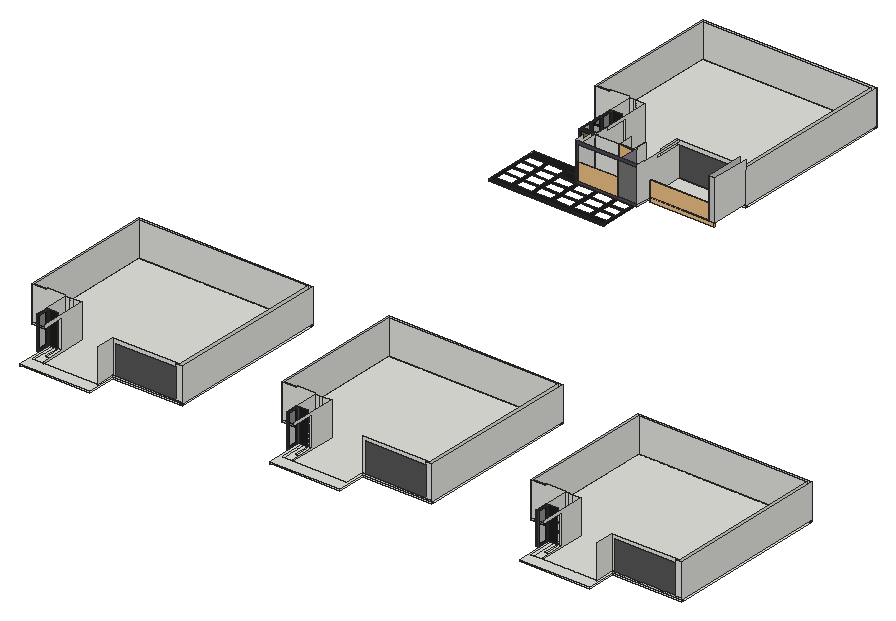
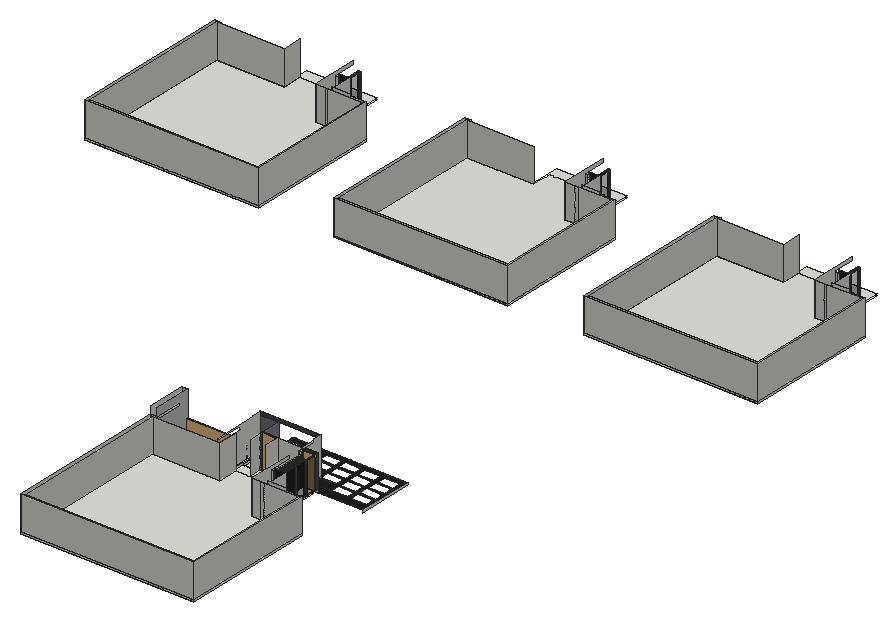
# SketchUp Ruby script. Lengths in inches.
U = 1.inch
M = Sketchup.active_model
def pt(a) = Geom::Point3d.new(a.map { |v| v * U })
def face(e, loops, mat)
  f = e.add_face(loops[0].map { |a| pt(a) })
  loops[1..].each { |l| e.add_face(l.map { |a| pt(a) }).erase! }
  f.material = f.back_material = mat if mat
  f
end
# faces: each face lists its corners as indices into pts; further lists are holes
def faces(e, pts, list, mat = nil) = list.each { |f| face(e, (f[0].is_a?(Array) ? f : [f]).map { |l| l.map { |i| pts[i] } }, mat) }
# xy, xz, yz: faces in a plane at the given z, y or x. An outline is a flat list of corners, or four numbers for a rectangle; further outlines are holes
def ring(l) = l.size == 4 ? [[l[0], l[1]], [l[2], l[1]], [l[2], l[3]], [l[0], l[3]]] : l.each_slice(2).to_a
def flat(e, list, mat, &to3) = list.each { |f| face(e, (f[0].is_a?(Array) ? f : [f]).map { |l| ring(l).map { |u, v| to3.(u, v) } }, mat) }
def xy(e, z, list, mat = nil) = flat(e, list, mat) { |x, y| [x, y, z] }
def xz(e, y, list, mat = nil) = flat(e, list, mat) { |x, z| [x, y, z] }
def yz(e, x, list, mat = nil) = flat(e, list, mat) { |y, z| [x, y, z] }
def lines(e, pts, list) = list.each { |a, b| e.add_line(pt(pts[a]), pt(pts[b])) }
# prism: a flat outline (further loops are holes) pulled along v
def prism(e, loops, v, mat = nil)
  f = face(e, loops, mat); d = Geom::Vector3d.new(v.map { |x| x * U })
  f.pushpull(f.normal.samedirection?(d) ? d.length : -d.length)
end
def box(e, o, s, mat = nil) = prism(e, [[o, [o[0] + s[0], o[1], o[2]], [o[0] + s[0], o[1] + s[1], o[2]], [o[0], o[1] + s[1], o[2]]]], [0, 0, s[2]], mat)
def at(x, y, z, deg = 0) = Geom::Transformation.translation(pt([x, y, z])) * Geom::Transformation.rotation(ORIGIN, Z_AXIS, deg.degrees)
def axes(o, x, y, z) = Geom::Transformation.new([*x, 0, *y, 0, *z, 0, *pt(o).to_a, 1])
def part(name) = M.definitions.add(name)
# library, detail: a bought-in or finely detailed component or shape, given as its bounding box
def library(name, o, s) = part(name).tap { |d| box(d.entities, o, s) }
def detail(e, o, s) = box(e.add_group.entities, o, s)
def put(e, d, t, mat = nil) = e.add_instance(d, t).tap { |i| i.material = mat if mat }
def group(e, t, mat = nil) = e.add_group.tap { |g| g.transformation = t; g.material = mat if mat }.entities
root = M.entities
M.materials.add("Glass_Tinted_Gray").color = [0, 0, 0]
M.materials["Glass_Tinted_Gray"].alpha = 0.125
M.materials.add("[0135_DarkGray]").color = [81, 81, 81]
M.materials.add("[Color M02]").color = [198, 198, 198]
M.materials.add("[Color M04]").color = [60, 133, 34]
M.materials.add("[Color M05]1").color = [114, 114, 114]
M.materials.add("[Color M06]").color = [79, 71, 84]
M.materials.add("[Color M06]1").color = [86, 86, 86]
M.materials.add("[Color M07]").color = [58, 58, 58]
M.materials.add("[Color M08]").color = [30, 30, 30]
M.materials.add("[Formica Graystone]1").color = [140, 132, 147]
M.materials.add("[Mirror 02]").color = [229, 229, 229]
c1 = part("PENTEK_RP Fineline 50S_SlidingDoor_Glass")
box(c1.entities,[0,0,0],[46.58,0.16,94.39],"Glass_Tinted_Gray")
c2 = part("PENTEK_RP Fineline 50S_SlidingDoor_GlazingBead")
box(c2.entities,[0,0,0],[45.47,0.59,0.56],"[0135_DarkGray]")
c3 = part("PENTEK_RP Fineline 50S_SlidingDoor_GlazingBead_2")
box(c3.entities,[0,0,0],[0.56,0.59,94.39],"[0135_DarkGray]")
c4 = part("PENTEK_RP Fineline 50S_SlidingDoor_Leaf_E1")
xy(c4.entities,0,[[0,0,0.93,1.97],[0.93,1.57,1.49,1.97]],"[0135_DarkGray]")
xy(c4.entities,96.25,[[0,0,0.93,0,0.93,1.57,1.49,1.57,1.49,1.97,0,1.97]],"[0135_DarkGray]")
xz(c4.entities,0,[[0,0,0.93,96.25]],"[0135_DarkGray]")
xz(c4.entities,1.57,[[0.93,0,1.49,95.32],[0.93,95.32,1.49,96.25]],"[0135_DarkGray]")
xz(c4.entities,1.97,[[0,0,1.49,96.25]],"[0135_DarkGray]")
yz(c4.entities,0,[[0,0,1.97,96.25]],"[0135_DarkGray]")
yz(c4.entities,0.93,[[0,0,1.57,0.93],[0,0.93,1.57,95.32],[0,95.32,1.57,96.25]],"[0135_DarkGray]")
yz(c4.entities,1.49,[[1.57,0,1.97,95.32],[1.57,95.32,1.97,96.25]],"[0135_DarkGray]")
c5 = part("PENTEK_RP Fineline 50S_SlidingDoor_Leaf_E2")
xy(c5.entities,0,[[0,0,0,1.57,0.56,1.57,0.56,1.97,46.02,1.97,46.02,1.57,46.58,1.57,46.58,0]],"[0135_DarkGray]")
xy(c5.entities,0.93,[[0,0,46.58,1.57]],"[0135_DarkGray]")
xy(c5.entities,1.49,[[0.56,1.57,46.02,1.97]],"[0135_DarkGray]")
xz(c5.entities,0,[[0,0,46.58,0.93]],"[0135_DarkGray]")
xz(c5.entities,1.57,[[0,0,0.56,0.93],[46.02,0,46.58,0.93],[0.56,0.93,46.02,1.49]],"[0135_DarkGray]")
xz(c5.entities,1.97,[[0.56,0,46.02,1.49]],"[0135_DarkGray]")
yz(c5.entities,0,[[0,0,1.57,0.93]],"[0135_DarkGray]")
yz(c5.entities,0.56,[[1.57,0,1.97,0.93],[1.57,0.93,1.97,1.49]],"[0135_DarkGray]")
yz(c5.entities,46.02,[[1.57,0,1.97,0.93],[1.57,0.93,1.97,1.49]],"[0135_DarkGray]")
yz(c5.entities,46.58,[[0,0,1.57,0.93]],"[0135_DarkGray]")
c6 = part("PENTEK_RP Fineline 50S_SlidingDoor_Leaf2")
put(c6.entities,c1,at(1.49,1.42,0.93))
put(c6.entities,c2,at(1.49,0,94.77))
put(c6.entities,c3,at(46.96,0,0.93))
put(c6.entities,c1,at(1.49,0.59,0.93),"[Mirror 02]")
put(c6.entities,c3,at(0.93,0,0.93))
put(c6.entities,c4,at(0,0,0))
put(c6.entities,c4,axes([48.44,0,0],[-1,0,0],[0,1,0],[0,0,1]))
put(c6.entities,c2,at(1.49,0,0.93))
put(c6.entities,c5,axes([0.93,0,96.25],[1,0,0],[0,1,0],[0,0,-1]))
put(c6.entities,c5,at(0.93,0,0))
c7 = part("glass-railing")
detail(c7.entities,[0,0,0],[1.26,75.59,33.1875])
c8 = library("Sliding Gate",[0,0,0],[194.88,4.13,70.58])
c9 = library("Aluprof_MB-86_Drzwi_panelowe_003_S-0452",[0,0,0],[44.84,5.36,87])
c10 = library("Group\#1",[0,0,0],[29.75,5.78,110.95])
xy(root,117.06,[[782.875,2157.49,1189.95,2158.62],[1189.64,2158.62,1189.95,2339.31]])
xy(root,123.92,[[1137.16,2157.49,1189.95,2158.62],[1189.64,2158.62,1189.95,2339.31]])
xy(root,123.92,[[782.875,2157.49,992.47,2158.62],[992.47,2157.49,1137.16,2158.62]],"[Color M08]")
xy(root,125.0625,[[429.58,521.5625,435.61,521.5625,435.61,732.16,312.24,732.16,312.24,1195.84,923.77,1195.84,923.77,1201.875,306.21,1201.875,306.21,726.125,429.58,726.125],[435.61,521.5625,677.53,521.5625,677.53,829.91,671.5,829.91,671.5,807.47,435.61,807.47],[1316.04,521.5625,1322.08,521.5625,1322.08,732.16,1198.7,732.16,1198.7,1195.84,1810.23,1195.84,1810.23,1201.875,1192.67,1201.875,1192.67,726.125,1316.04,726.125],[1322.08,521.5625,1563.99,521.5625,1563.99,829.91,1557.96,829.91,1557.96,807.47,1322.08,807.47],[2202.51,521.5625,2208.54,521.5625,2208.54,732.16,2085.16,732.16,2085.16,1195.84,2696.7,1195.84,2696.7,1201.875,2079.13,1201.875,2079.13,726.125,2202.51,726.125],
  [2208.54,521.5625,2450.46,521.5625,2450.46,829.91,2444.43,829.91,2444.43,807.47,2208.54,807.47],[677.53,623.84,923.77,623.84,923.77,629.875,908.11,629.875,908.11,829.91,677.53,829.91],[1563.99,623.84,1810.23,623.84,1810.23,629.875,1794.58,629.875,1794.58,829.91,1563.99,829.91],[2450.46,623.84,2696.7,623.84,2696.7,629.875,2681.04,629.875,2681.04,829.91,2450.46,829.91],[908.11,629.875,923.77,1195.84],
  [1794.58,629.875,1810.23,1195.84],[2681.04,629.875,2696.7,1195.84],[312.24,732.16,312.24,1195.84,908.11,1195.84,908.11,829.91,671.5,829.91,671.5,807.47,435.61,807.47,435.61,732.16],[1198.7,732.16,1198.7,1195.84,1794.58,1195.84,1794.58,829.91,1557.96,829.91,1557.96,807.47,1322.08,807.47,1322.08,732.16],[2085.16,732.16,2085.16,1195.84,2681.04,1195.84,2681.04,829.91,2444.43,829.91,2444.43,807.47,2208.54,807.47,2208.54,732.16],
  [986.75,2289.06,986.75,2293.87,989.57,2293.87,989.57,2327.31,986.75,2327.31,986.75,2373.56,992.47,2373.56,992.47,2289.06],[[992.47,2289.06,1137.16,2373.56],[1000.51,2293.87,1058.47,2327.31],[1069.4,2294.18,1127.36,2327.31]],[[1137.16,2289.06,1137.16,2373.56,1196.26,2373.56,1196.26,2339.31,1189.95,2339.31,1189.95,2289.06],[1138.3,2293.85,1187.76,2327.31]],[1189.95,2289.06,1205.57,2339.31],[986.75,2293.87,989.57,2327.31],
  [948.3125,2373.56,954.34,2373.56,954.34,2584.15,830.97,2584.15,830.97,3047.84,1442.5,3047.84,1442.5,3053.87,824.9375,3053.87,824.9375,2578.12,948.3125,2578.12],[954.34,2373.56,1196.26,2373.56,1196.26,2681.9,1190.23,2681.9,1190.23,2659.46,954.34,2659.46],[1196.26,2475.84,1442.5,2475.84,1442.5,2481.87,1426.84,2481.87,1426.84,2681.9,1196.26,2681.9],[1426.84,2481.87,1442.5,3047.84],[830.97,2584.15,830.97,3047.84,1426.84,3047.84,1426.84,2681.9,1190.23,2681.9,1190.23,2659.46,954.34,2659.46,954.34,2584.15]])
xy(root,125.0625,[[[782.875,2157.49,1189.95,2289.06],[862.71,2253.62,920.67,2287.85],[931.61,2253.62,989.57,2287.85],[1000.51,2253.62,1058.47,2287.85],[1069.4,2253.74,1127.36,2287.85],[862.71,2214.37,920.67,2248.4],[931.61,2214.37,989.57,2248.4],[1000.51,2214.37,1058.47,2248.4],[794.625,2253.62,851.77,2287.85],[794.625,2214.37,851.77,2248.4],[1069.4,2214.87,1127.36,2248.4],[862.71,2175.49,920.67,2208.95],[931.61,2175.49,989.57,2208.95],[1000.51,2175.49,1058.47,2208.95],[1069.4,2175.49,1127.36,2208.95],[794.625,2175.49,851.77,2208.95],[1138.3,2254.4,1187.76,2287.85],[1138.3,2214.95,1187.76,2248.4],[1138.3,2175.49,1187.76,2208.95]],[[782.875,2289.06,986.75,2289.06,986.75,2293.87,931.61,2293.87,931.61,2327.31,986.75,2327.31,986.75,2357.31,782.875,2357.31],[862.71,2293.87,920.67,2327.31],[794.625,2293.87,851.77,2327.31]],[931.61,2293.87,986.75,2327.31]],"[Color M08]")
xy(root,131.0625,[[[429.58,521.5625,429.58,726.125,306.21,726.125,306.21,1201.875,923.77,1201.875,923.77,623.84,677.53,623.84,677.53,521.5625],[435.78,561.375,446.59,561.375,446.59,562.32,671.33,562.32,671.33,630.04,910.57,630.04,910.57,1195.68,312.41,1195.68,312.41,732.32,435.78,732.32]],[[1316.04,521.5625,1316.04,726.125,1192.67,726.125,1192.67,1201.875,1810.23,1201.875,1810.23,623.84,1563.99,623.84,1563.99,521.5625],[1322.24,561.375,1333.06,561.375,1333.06,562.32,1557.79,562.32,1557.79,630.04,1797.03,630.04,1797.03,1195.68,1198.87,1195.68,1198.87,732.32,1322.24,732.32]],[[2202.51,521.5625,2202.51,726.125,2079.13,726.125,2079.13,1201.875,2696.7,1201.875,2696.7,623.84,2450.46,623.84,2450.46,521.5625],[2208.71,561.375,2219.52,561.375,2219.52,562.32,2444.26,562.32,2444.26,630.04,2683.5,630.04,2683.5,1195.68,2085.33,1195.68,2085.33,732.32,2208.71,732.32]],[478.78,562.32,671.33,562.32,671.33,630.04,910.57,630.04,910.57,1195.68,312.41,1195.68,312.41,732.32,478.78,732.32],[435.78,562.32,446.59,732.32],
  [446.59,562.32,478.78,732.32],[1365.24,562.32,1557.79,562.32,1557.79,630.04,1797.03,630.04,1797.03,1195.68,1198.87,1195.68,1198.87,732.32,1365.24,732.32],[1322.24,562.32,1333.06,732.32],[1333.06,562.32,1365.24,732.32],[2251.71,562.32,2444.26,562.32,2444.26,630.04,2683.5,630.04,2683.5,1195.68,2085.33,1195.68,2085.33,732.32,2251.71,732.32],
  [2208.71,562.32,2219.52,732.32],[2219.52,562.32,2251.71,732.32],[[948.3125,2373.56,948.3125,2578.12,824.9375,2578.12,824.9375,3053.87,1442.5,3053.87,1442.5,2475.84,1196.26,2475.84,1196.26,2373.56],[954.51,2413.37,965.32,2413.37,965.32,2414.32,1190.0625,2414.32,1190.0625,2482.04,1429.3,2482.04,1429.3,3047.67,831.14,3047.67,831.14,2584.32,954.51,2584.32]],[954.51,2413.37,965.32,2414.32],[997.51,2414.32,1190.0625,2414.32,1190.0625,2482.04,1429.3,2482.04,1429.3,3047.67,831.14,3047.67,831.14,2584.32,997.51,2584.32],
  [954.51,2414.32,965.32,2584.32],[965.32,2414.32,997.51,2584.32]])
xy(root,135.875,[[997.28,2289.06,1137.16,2289.06,1137.16,2373.56,1083.76,2373.56,1083.76,2361.68,997.28,2361.68],[997.28,2361.68,1083.76,2373.56],[1083.76,2373.56,1137.16,2414.32]])
xy(root,136.125,[[463.64,591.8125,468.02,646.3125],[468.02,591.8125,478.78,646.3125],[1350.1,591.8125,1354.48,646.3125],[1354.48,591.8125,1365.24,646.3125],[2236.57,591.8125,2240.94,646.3125],
  [2240.94,591.8125,2251.71,646.3125],[424.39,646.3125,445.77,686.3125],[1310.86,646.3125,1332.23,686.3125],[2197.32,646.3125,2218.7,686.3125],[1196.26,2339.31,1205.57,2373.56],
  [1205.57,2339.31,1419.96,2475.84],[1419.96,2339.31,1442.5,2475.84],[943.125,2357.31,982.37,2498.31],[982.37,2357.31,986.75,2414.32],[1196.26,2373.56,1205.57,2475.84],
  [982.37,2414.32,986.75,2443.81],[986.75,2414.32,997.51,2443.81],[982.37,2443.81,986.75,2498.31],[986.75,2443.81,997.51,2498.31],[943.125,2498.31,964.5,2538.31]])
xz(root,623.84,[[677.53,131.0625,923.77,136.125],[1563.99,131.0625,1810.23,136.125],[2450.46,131.0625,2696.7,136.125],[901.22,136.125,923.77,251.0625],[1787.6875,136.125,1810.23,251.0625],
  [2674.15,136.125,2696.7,251.0625]])
xz(root,623.84,[[686.84,136.125,901.22,240.88],[1573.31,136.125,1787.6875,240.88],[2459.77,136.125,2674.15,240.88]],"[Color M06]1")
xz(root,630.04,[[671.33,131.0625,910.57,251.0625],[1557.79,131.0625,1797.03,251.0625],[2444.26,131.0625,2683.5,251.0625]])
xz(root,646.3125,[[463.64,136.125,468.02,240.47],[468.02,136.125,478.78,240.47],[1350.1,136.125,1354.48,240.47],[1354.48,136.125,1365.24,240.47],[2236.57,136.125,2240.94,240.47],
  [2240.94,136.125,2251.71,240.47]])
xz(root,646.3125,[[424.39,136.125,463.64,251.0625],[1310.86,136.125,1350.1,251.0625],[2197.32,136.125,2236.57,251.0625]],"[Color M08]")
xz(root,726.125,[[306.21,125.0625,424.39,131.0625],[1192.67,125.0625,1310.86,131.0625],[2079.13,125.0625,2197.32,131.0625],[306.21,131.0625,424.39,131.0625,424.39,258.95,363.02,258.95,363.02,251.0625,306.21,251.0625],[424.39,131.0625,429.58,136.125],
  [1192.67,131.0625,1310.86,131.0625,1310.86,258.95,1249.48,258.95,1249.48,251.0625,1192.67,251.0625],[1310.86,131.0625,1316.04,136.125],[2079.13,131.0625,2197.32,131.0625,2197.32,258.95,2135.95,258.95,2135.95,251.0625,2079.13,251.0625],[2197.32,131.0625,2202.51,136.125]])
xz(root,732.32,[[312.41,131.0625,435.78,251.0625],[435.78,131.0625,446.59,251.0625],[446.59,131.0625,478.78,251.0625],[1198.87,131.0625,1322.24,251.0625],[1322.24,131.0625,1333.06,251.0625],
  [1333.06,131.0625,1365.24,251.0625],[2085.33,131.0625,2208.71,251.0625],[2208.71,131.0625,2219.52,251.0625],[2219.52,131.0625,2251.71,251.0625]])
xz(root,1195.68,[[312.41,131.0625,910.57,251.0625],[1198.87,131.0625,1797.03,251.0625],[2085.33,131.0625,2683.5,251.0625]])
xz(root,1201.875,[[306.21,125.0625,923.77,131.0625],[1192.67,125.0625,1810.23,131.0625],[2079.13,125.0625,2696.7,131.0625],[306.21,131.0625,923.77,251.0625],[1192.67,131.0625,1810.23,251.0625],
  [2079.13,131.0625,2696.7,251.0625]])
xz(root,2157.49,[[782.875,123.92,1189.95,125.0625]],"[Color M08]")
xz(root,2158.62,[[782.875,117.06,1189.64,123.92]],"[Color M08]")
xz(root,2289.06,[[1137.16,135.875,1205.57,251.0625]],"[Color M05]1")
xz(root,2289.06,[[986.75,125.0625,1205.57,125.0625,1205.57,135.875,997.28,135.875,997.28,250.875,1137.16,250.875,1137.16,251.0625,1205.57,251.0625,1205.57,263.89,986.75,263.89]],"[Color M06]")
xz(root,2339.31,[[1196.26,125.0625,1205.57,131.0625],[1196.26,131.0625,1205.57,136.125]])
xz(root,2339.31,[[1419.96,136.125,1442.5,278.1875]],"[Color M02]")
xz(root,2357.31,[[943.125,125.0625,986.75,136.125],[982.37,136.125,986.75,240.47]])
xz(root,2361.68,[[997.28,135.875,1083.76,250.875]])
xz(root,2373.56,[[986.75,125.0625,992.47,131.0625],[992.47,125.0625,1137.16,131.0625],[1137.16,125.0625,1196.26,131.0625],[986.75,131.0625,992.47,251.0625],[992.47,131.0625,997.28,246.25],
  [997.28,131.0625,1137.16,135.875]])
xz(root,2475.84,[[1196.26,131.0625,1442.5,136.125],[1419.96,136.125,1442.5,251.0625]])
xz(root,2475.84,[[1205.57,136.125,1419.96,240.88]],"[Color M06]1")
xz(root,2482.04,[[1190.0625,131.0625,1429.3,251.0625]])
xz(root,2498.31,[[982.37,136.125,986.75,240.47],[986.75,136.125,997.51,240.47]])
xz(root,2498.31,[[943.125,136.125,982.37,251.0625]],"[Color M08]")
xz(root,2578.12,[[824.9375,125.0625,943.125,131.0625],[824.9375,131.0625,943.125,131.0625,943.125,258.95,881.75,258.95,881.75,251.0625,824.9375,251.0625],[943.125,131.0625,948.3125,136.125]])
xz(root,2584.32,[[831.14,131.0625,954.51,251.0625],[954.51,131.0625,965.32,251.0625],[965.32,131.0625,997.51,251.0625]])
xz(root,3047.67,[[831.14,131.0625,1429.3,251.0625]])
xz(root,3053.87,[[824.9375,125.0625,1442.5,131.0625],[824.9375,131.0625,1442.5,251.0625]])
yz(root,306.21,[[726.125,125.0625,1201.875,131.0625],[726.125,131.0625,1201.875,251.0625]])
yz(root,312.41,[[732.32,131.0625,1195.68,251.0625]])
yz(root,424.39,[[646.3125,136.125,726.125,251.0625]])
yz(root,478.78,[[562.32,131.0625,732.32,131.0625,732.32,251.0625,567.01,251.0625,567.01,240.47,646.3125,240.47,646.3125,136.125,562.32,136.125]])
yz(root,671.33,[[562.32,131.0625,630.04,251.0625]])
yz(root,782.875,[[2157.49,117.06,2158.62,117.65],[2157.49,117.65,2158.62,123.92],[2158.62,117.65,2158.62,123.92,2157.49,123.92,2157.49,125.0625,2357.31,125.0625,2357.31,117.65]])
yz(root,824.9375,[[2578.12,125.0625,3053.87,131.0625],[2578.12,131.0625,3053.87,251.0625]])
yz(root,831.14,[[2584.32,131.0625,3047.67,251.0625]])
yz(root,910.57,[[630.04,131.0625,1195.68,251.0625]])
yz(root,923.77,[[623.84,131.0625,1201.875,251.0625]])
yz(root,943.125,[[2498.31,136.125,2578.12,251.0625]])
yz(root,954.51,[[2413.37,131.0625,2414.32,136.125]])
yz(root,982.37,[[2357.31,136.125,2498.31,240.47]],"[Color M07]")
yz(root,986.75,[[2289.06,125.0625,2357.31,131.0625],[2357.31,125.0625,2373.56,136.125],[2289.06,131.0625,2289.06,263.89,2321.87,263.89,2321.87,251.0625,2357.31,251.0625,2357.31,131.0625],[2357.31,136.125,2373.56,240.47],[2373.56,136.125,2498.31,240.47]])
yz(root,997.28,[[2289.06,135.875,2361.68,250.875],[2361.68,135.875,2373.56,246.25]])
yz(root,997.51,[[2414.32,131.0625,2584.32,131.0625,2584.32,251.0625,2419.01,251.0625,2419.01,240.47,2498.31,240.47,2498.31,136.125,2414.32,136.125]])
yz(root,1083.76,[[2361.68,135.875,2414.32,135.875,2414.32,251.0625,2373.56,251.0625,2373.56,250.875,2361.68,250.875]])
yz(root,1137.16,[[2373.56,135.875,2414.32,251.0625]])
yz(root,1137.16,[[2289.06,135.875,2373.56,250.875]],"[Formica Graystone]1")
yz(root,1189.64,[[2158.62,117.06,2339.31,123.92]],"[Color M08]")
yz(root,1189.95,[[2157.49,123.92,2339.31,125.0625]],"[Color M08]")
yz(root,1190.0625,[[2414.32,131.0625,2482.04,251.0625]])
yz(root,1192.67,[[726.125,125.0625,1201.875,131.0625],[726.125,131.0625,1201.875,251.0625]])
yz(root,1196.26,[[2339.31,125.0625,2373.56,131.0625],[2339.31,131.0625,2373.56,136.125],[2373.56,131.0625,2475.84,136.125]])
yz(root,1198.87,[[732.32,131.0625,1195.68,251.0625]])
yz(root,1205.57,[[2289.06,125.0625,2339.31,131.0625],[2289.06,131.0625,2339.31,131.0625,2339.31,136.125,2475.84,136.125,2475.84,240.88,2373.56,240.88,2373.56,242.34,2374.81,242.34,2374.81,249.61,2373.56,249.61,2373.56,251.0625,2475.84,251.0625,2475.84,257.0625,2319.18,257.0625,2319.18,258.95,2289.06,258.95]])
yz(root,1310.86,[[646.3125,136.125,726.125,251.0625]])
yz(root,1365.24,[[562.32,131.0625,732.32,131.0625,732.32,251.0625,567.01,251.0625,567.01,240.47,646.3125,240.47,646.3125,136.125,562.32,136.125]])
yz(root,1419.96,[[2339.31,136.125,2339.31,278.1875,2475.84,278.1875,2475.84,251.0625,2373.56,251.0625,2373.56,249.61,2374.81,249.61,2374.81,242.34,2373.56,242.34,2373.56,240.88,2475.84,240.88,2475.84,136.125]],"[Color M02]")
yz(root,1429.3,[[2482.04,131.0625,3047.67,251.0625]])
yz(root,1442.5,[[2475.84,131.0625,3053.87,251.0625],[2339.31,136.125,2475.84,278.1875]])
yz(root,1797.03,[[630.04,131.0625,1195.68,251.0625]])
yz(root,1810.23,[[623.84,131.0625,1201.875,251.0625]])
yz(root,2079.13,[[726.125,125.0625,1201.875,131.0625],[726.125,131.0625,1201.875,251.0625]])
yz(root,2085.33,[[732.32,131.0625,1195.68,251.0625]])
yz(root,2197.32,[[646.3125,136.125,726.125,251.0625]])
yz(root,2251.71,[[562.32,131.0625,732.32,131.0625,732.32,251.0625,567.01,251.0625,567.01,240.47,646.3125,240.47,646.3125,136.125,562.32,136.125]])
yz(root,2444.26,[[562.32,131.0625,630.04,251.0625]])
yz(root,2683.5,[[630.04,131.0625,1195.68,251.0625]])
yz(root,2696.7,[[623.84,131.0625,1201.875,251.0625]])
p = [[997.28,2373.56,131.0625],[997.28,2319.18,131.0625],[992.47,2373.56,131.0625],[992.47,2319.18,131.0625],[948.3125,2373.56,131.0625],[948.3125,2373.56,136.125]]
lines(root,p,[[0,1],[2,3],[4,5]])
put(root,c6,axes([1310.86,644.6,136.125],[0,-0.90045,0],[3.85,0,0],[0,0,1.1941]))
put(root,c6,axes([2197.32,644.6,136.125],[0,-0.90045,0],[3.85,0,0],[0,0,1.1941]))
put(root,c6,axes([424.39,644.6,136.125],[0,-0.90045,0],[3.85,0,0],[0,0,1.1941]))
put(root,c7,axes([997.28,2289.06,135.875],[0,-1.85,0],[1.85,0,0],[0,0,1.85]))
put(root,c8,axes([1205.57,2343.02,118.7],[1.17982,0,0],[0,1,0],[0,0,1]))
put(root,c6,axes([943.125,2357.31,136.125],[0.90045,0,0],[0,3.85,0],[0,0,1.1941]))
put(root,c9,axes([1083.76,2360.77,135.875],[1.16659,-0.08923,0],[0.08923,1.16659,0],[0,0,1.32399]))
put(root,c10,axes([943.125,2367.62,136.125],[1.38276,0,0],[0,1,0],[0,0,1.03593]),"[Color M04]")
put(root,c6,axes([943.13,2408.51,136.125],[0,-0.90045,0],[0.924,0,0],[0,0,1.1941]))
put(root,c6,axes([943.125,2452.13,136.125],[0,-0.90045,0],[3.85,0,0],[0,0,1.1941]))
put(root,c6,axes([943.125,2496.59,136.125],[0,-0.90045,0],[3.85,0,0],[0,0,1.1941]))
